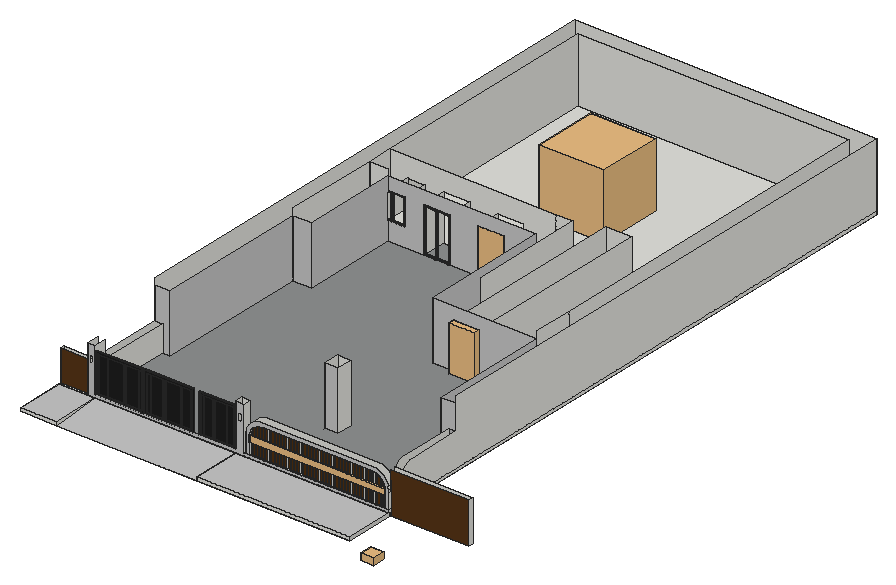
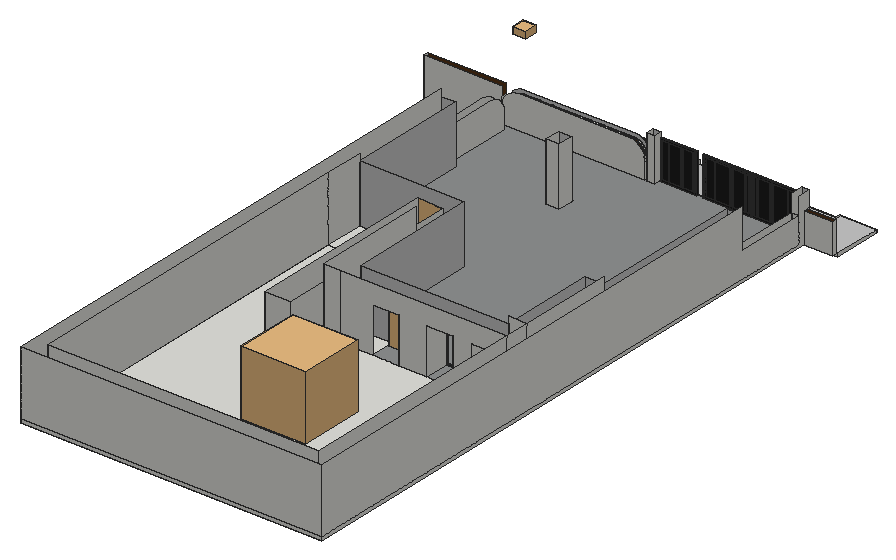
# SketchUp Ruby script. Lengths in inches.
U = 1.inch
M = Sketchup.active_model
def pt(a) = Geom::Point3d.new(a.map { |v| v * U })
def face(e, loops, mat)
  f = e.add_face(loops[0].map { |a| pt(a) })
  loops[1..].each { |l| e.add_face(l.map { |a| pt(a) }).erase! }
  f.material = f.back_material = mat if mat
  f
end
# faces: each face lists its corners as indices into pts; further lists are holes
def faces(e, pts, list, mat = nil) = list.each { |f| face(e, (f[0].is_a?(Array) ? f : [f]).map { |l| l.map { |i| pts[i] } }, mat) }
# xy, xz, yz: faces in a plane at the given z, y or x. An outline is a flat list of corners, or four numbers for a rectangle; further outlines are holes
def ring(l) = l.size == 4 ? [[l[0], l[1]], [l[2], l[1]], [l[2], l[3]], [l[0], l[3]]] : l.each_slice(2).to_a
def flat(e, list, mat, &to3) = list.each { |f| face(e, (f[0].is_a?(Array) ? f : [f]).map { |l| ring(l).map { |u, v| to3.(u, v) } }, mat) }
def xy(e, z, list, mat = nil) = flat(e, list, mat) { |x, y| [x, y, z] }
def xz(e, y, list, mat = nil) = flat(e, list, mat) { |x, z| [x, y, z] }
def yz(e, x, list, mat = nil) = flat(e, list, mat) { |y, z| [x, y, z] }
def lines(e, pts, list) = list.each { |a, b| e.add_line(pt(pts[a]), pt(pts[b])) }
# prism: a flat outline (further loops are holes) pulled along v
def prism(e, loops, v, mat = nil)
  f = face(e, loops, mat); d = Geom::Vector3d.new(v.map { |x| x * U })
  f.pushpull(f.normal.samedirection?(d) ? d.length : -d.length)
end
def box(e, o, s, mat = nil) = prism(e, [[o, [o[0] + s[0], o[1], o[2]], [o[0] + s[0], o[1] + s[1], o[2]], [o[0], o[1] + s[1], o[2]]]], [0, 0, s[2]], mat)
def at(x, y, z, deg = 0) = Geom::Transformation.translation(pt([x, y, z])) * Geom::Transformation.rotation(ORIGIN, Z_AXIS, deg.degrees)
def axes(o, x, y, z) = Geom::Transformation.new([*x, 0, *y, 0, *z, 0, *pt(o).to_a, 1])
def part(name) = M.definitions.add(name)
# library, detail: a bought-in or finely detailed component or shape, given as its bounding box
def library(name, o, s) = part(name).tap { |d| box(d.entities, o, s) }
def detail(e, o, s) = box(e.add_group.entities, o, s)
def put(e, d, t, mat = nil) = e.add_instance(d, t).tap { |i| i.material = mat if mat }
def group(e, t, mat = nil) = e.add_group.tap { |g| g.transformation = t; g.material = mat if mat }.entities
root = M.entities
M.materials.add("Wine2").color = [0, 0, 0]
M.materials["Wine2"].alpha = 0
M.materials.add("[0130_Gainsboro]").color = [39, 45, 50]
M.materials.add("[Blacktop Old 02]").color = [143, 145, 145]
M.materials.add("[Color M02]").color = [198, 198, 198]
M.materials.add("[Color M08]1").color = [30, 30, 30]
M.materials.add("[Wood Floor Dark]").color = [86, 53, 23]
M.materials.add("[Wood Square Tile 02]").color = [81, 47, 16]
c1 = library("door (1)",[38.93,25.48,0],[40,9.94,82.68])
c2 = part("Framed glazing panel")
xy(c2.entities,0,[[0,-0.98,43.07,0],[0,0,43.07,1.4]],"[0130_Gainsboro]")
xy(c2.entities,0.3,[[0.3,-1.43,42.77,-0.98]],"[0130_Gainsboro]")
xy(c2.entities,2.95,[[2.95,-1.43,40.12,-0.63],[2.95,-0.63,40.12,0],[2.95,0,40.12,0.64],[2.95,0.64,40.12,1.4]],"[0130_Gainsboro]")
xy(c2.entities,3.54,[[3.54,-0.63,39.53,0],[3.54,0,39.53,0.64]],"[0130_Gainsboro]")
xy(c2.entities,111.8125,[[3.54,-0.63,39.53,0],[3.54,0,39.53,0.64]],"[0130_Gainsboro]")
xy(c2.entities,112.4,[[2.95,-1.43,40.12,-0.63],[2.95,-0.63,40.12,0],[2.95,0,40.12,0.64],[2.95,0.64,40.12,1.4]],"[0130_Gainsboro]")
xy(c2.entities,115.05,[[0.3,-1.43,42.77,-0.98]],"[0130_Gainsboro]")
xy(c2.entities,115.35,[[0,-0.98,43.07,0],[0,0,43.07,1.4]],"[0130_Gainsboro]")
xz(c2.entities,-1.43,[[[0.3,0.3,42.77,115.05],[2.95,2.95,40.12,112.4]]],"[0130_Gainsboro]")
xz(c2.entities,-0.98,[[[0,0,43.07,115.35],[0.3,0.3,42.77,115.05]]],"[0130_Gainsboro]")
xz(c2.entities,-0.63,[[[2.95,2.95,40.12,112.4],[3.54,3.54,39.53,111.8125]]],"[0130_Gainsboro]")
xz(c2.entities,0,[[3.54,3.54,39.53,111.8125]],"Wine2")
xz(c2.entities,0,[[[0,0,43.07,115.35],[2.95,2.95,40.12,112.4]],[[2.95,2.95,40.12,112.4],[3.54,3.54,39.53,111.8125]]],"[0130_Gainsboro]")
xz(c2.entities,0.64,[[[2.95,2.95,40.12,112.4],[3.54,3.54,39.53,111.8125]]],"[0130_Gainsboro]")
xz(c2.entities,1.4,[[[0,0,43.07,115.35],[2.95,2.95,40.12,112.4]]],"[0130_Gainsboro]")
yz(c2.entities,0,[[-0.98,0,0,115.35],[0,0,1.4,115.35]],"[0130_Gainsboro]")
yz(c2.entities,0.3,[[-1.43,0.3,-0.98,115.05]],"[0130_Gainsboro]")
yz(c2.entities,2.95,[[-1.43,2.95,-0.63,112.4],[-0.63,2.95,0,112.4],[0,2.95,0.64,112.4],[0.64,2.95,1.4,112.4]],"[0130_Gainsboro]")
yz(c2.entities,3.54,[[-0.63,3.54,0,111.8125],[0,3.54,0.64,111.8125]],"[0130_Gainsboro]")
yz(c2.entities,39.53,[[-0.63,3.54,0,111.8125],[0,3.54,0.64,111.8125]],"[0130_Gainsboro]")
yz(c2.entities,40.12,[[-1.43,2.95,-0.63,112.4],[-0.63,2.95,0,112.4],[0,2.95,0.64,112.4],[0.64,2.95,1.4,112.4]],"[0130_Gainsboro]")
yz(c2.entities,42.77,[[-1.43,0.3,-0.98,115.05]],"[0130_Gainsboro]")
yz(c2.entities,43.07,[[-0.98,0,0,115.35],[0,0,1.4,115.35]],"[0130_Gainsboro]")
c3 = part("Group\#1")
put(c3.entities,c2,axes([45.29,1.43,0],[1.05148,0,0],[0,1,0],[0,0,1]))
put(c3.entities,c2,axes([0,1.43,0],[1.05148,0,0],[0,1,0],[0,0,1]))
c4 = part("Group\#102")
g1 = group(c4.entities,at(0,0,0))
prism(g1,[[[0,3,72],[70.5,3,72],[70.5,3,0],[0,3,0]],[[67.5,3,3],[67.5,3,69],[3,3,69],[3,3,3]]],[0,-3,0])
c5 = part("Group\#135")
box(c5.entities,[0,0,0],[0.5,1,66])
c6 = part("Group\#148")
box(c6.entities,[0,-1,0],[5.5,1,66])
box(c6.entities,[50.84,-1,0],[13.66,1,66])
box(c6.entities,[28.06,-1,0],[22.28,1,66])
box(c6.entities,[24.66,-1,0],[2.9,1,66])
box(c6.entities,[6,-1,0],[18.16,1,66])
c7 = part("Entrance gate assembly")
g2 = group(c7.entities,at(70.5,0,0),"[Color M08]1")
put(g2,c4,axes([70.5,0,0],[-1,0,0],[0,1,0],[0,0,1]))
g3 = group(g2,at(3,2,3))
g4 = group(g3,at(0,-1,0))
box(g4,[0,0,0],[5.5,1,66])
box(g4,[50.84,0,0],[13.66,1,66])
box(g4,[28.06,0,0],[22.28,1,66])
box(g4,[24.66,0,0],[2.9,1,66])
box(g4,[6,0,0],[18.16,1,66])
put(g3,c5,axes([50.34,0,0],[1,0,0],[0,-1,0],[0,0,1]))
put(g3,c5,axes([24.16,0,0],[1,0,0],[0,-1,0],[0,0,1]))
put(g3,c5,axes([27.56,0,0],[1,0,0],[0,-1,0],[0,0,1]))
put(g3,c5,axes([5.5,0,0],[1,0,0],[0,-1,0],[0,0,1]))
g5 = group(c7.entities,at(70.5,0,0),"[Color M08]1")
put(g5,c4,at(-70.5,0,0))
g6 = group(g5,at(-3,2,3,-180))
put(g6,c6,at(0,1,0))
put(g6,c5,at(50.34,0,0))
put(g6,c5,at(24.16,0,0))
put(g6,c5,at(27.56,0,0))
put(g6,c5,at(5.5,0,0))
g7 = group(c7.entities,at(150,0,0),"[Color M08]1")
put(g7,c4,axes([54,0,0],[-0.76596,0,0],[0,1,0],[0,0,1]))
g8 = group(g7,at(2.3,2,3))
put(g8,c6,axes([0,-1,0],[0.76596,0,0],[0,-1,0],[0,0,1]))
put(g8,c5,axes([38.55,0,0],[0.76596,0,0],[0,-1,0],[0,0,1]))
put(g8,c5,axes([18.5,0,0],[0.76596,0,0],[0,-1,0],[0,0,1]))
put(g8,c5,axes([21.11,0,0],[0.76596,0,0],[0,-1,0],[0,0,1]))
put(g8,c5,axes([4.22,0,0],[0.76596,0,0],[0,-1,0],[0,0,1]))
c8 = library("Omni Light",[-12,-12,-12],[24,24,24])
c9 = library("Mesh Light\#1",[-0.5,-0.5,-0.1],[1,1,0.2])
c10 = library("Dome Light",[-12,-12,0],[24,24,12])
xy(root,-12.28,[[0,0,326.57,89.5625],[326.57,0,609.5625,89.5625],[610.25,94.125,754.3125,104.0625]])
xy(root,-6,[[0,89.5625,52.9375,94.125],[52.9375,89.5625,52.9375,94.125,0,94.125,0,101.45,52.9375,101.45,52.9375,1217.1875,610.25,1217.1875,610.25,89.5625]])
xy(root,-6,[[0,0,66.8125,89.5625],[326.57,0,610.25,89.5625]],"[Color M02]")
xy(root,0,[[352.65,89.5625,354.44,92.0625],[354.44,89.5625,357.5,92.8125],[357.5,89.5625,361.83,92.0625],[361.83,89.5625,367.13,92.8125],[367.13,89.5625,373.05,92.0625],
  [373.05,89.5625,378.96,92.8125],[378.96,89.5625,384.88,92.0625],[384.88,89.5625,390.79,92.8125],[390.79,89.5625,396.71,92.0625],[396.71,89.5625,402.625,92.8125],
  [402.625,89.5625,408.54,92.0625],[408.54,89.5625,414.45,92.8125],[414.45,89.5625,420.37,92.0625],[420.37,89.5625,426.28,92.8125],[426.28,89.5625,432.2,92.0625],
  [432.2,89.5625,438.11,92.8125],[438.11,89.5625,444.03,92.0625],[444.03,89.5625,449.94,92.8125],[449.94,89.5625,455.86,92.0625],[455.86,89.5625,461.77,92.8125],
  [461.77,89.5625,467.6875,92.0625],[467.6875,89.5625,473.6,92.8125],[473.6,89.5625,479.52,92.0625],[479.52,89.5625,485.43,92.8125],[485.43,89.5625,491.35,92.0625],
  [491.35,89.5625,497.26,92.8125],[497.26,89.5625,503.18,92.0625],[503.18,89.5625,509.09,92.8125],[509.09,89.5625,515,92.0625],[515,89.5625,520.92,92.8125],
  [520.92,89.5625,526.83,92.0625],[526.83,89.5625,532.75,92.8125],[532.75,89.5625,538.66,92.0625],[538.66,89.5625,544.58,92.8125],[544.58,89.5625,550.49,92.0625],
  [550.49,89.5625,556.41,92.8125],[556.41,89.5625,562.32,92.0625],[562.32,89.5625,568.24,92.8125],[568.24,89.5625,572.45,92.0625],[572.45,89.5625,576.66,92.8125],
  [576.66,89.5625,581.24,92.0625],[581.24,89.5625,586.78,92.8125],[586.78,89.5625,592.76,92.0625],[592.76,89.5625,595.36,92.8125],[595.36,89.5625,599.57,92.0625],
  [599.57,89.5625,603.11,92.0625],[52.9375,113,66.86,113,66.86,244.9375,80.78,244.9375,80.78,1189.34,582.4,1189.34,582.4,244.9375,596.33,244.9375,596.33,115.8125,610.25,115.8125,610.25,1217.1875,52.9375,1217.1875],[388.8,467.53,427.3,467.53,427.3,539.85,420.8,539.85,420.8,752.85,329.63,752.85,329.63,706.78,388.8,706.78],[475.3,467.53,582.4,539.85],[420.8,539.85,427.3,539.85,427.3,820.03,475.3,820.03,475.3,539.85,582.4,539.85,582.4,1189.34,80.78,1189.34,80.78,752.85,420.8,752.85],
  [80.78,706.78,181,752.85],[229,706.78,281.63,752.85]])
xy(root,0,[[[66.86,89.5625,326.57,89.5625,326.57,104.75,341.76,104.75,341.76,89.5625,345.52,89.5625,345.52,104.0625,610.25,104.0625,610.25,115.8125,596.33,115.8125,596.33,244.9375,582.4,244.9375,582.4,467.53,475.3,467.53,475.3,820.03,427.3,820.03,427.3,467.53,388.8,467.53,388.8,706.78,329.63,706.78,329.63,752.85,281.63,752.85,281.63,706.78,229,706.78,229,752.85,181,752.85,181,706.78,115.1,706.78,115.1,529.39,80.78,529.39,80.78,244.9375,66.86,244.9375],[388.4375,219.25,412.5,248.6]]],"[Blacktop Old 02]")
xy(root,34.97,[[115.1,706.78,146.03,752.85]])
xz(root,0,[[0,-12.28,66.8125,-6],[326.57,-12.28,609.5625,-12.28,610.25,-6,326.57,-6]])
xz(root,89.5625,[[0,-12.28,326.57,-6],[326.57,-12.28,326.57,-6,610.25,-6,609.5625,-12.28]])
xz(root,89.5625,[[[52.9375,-6,610.25,-6,610.25,0,341.76,0,341.76,79.6875,326.57,79.6875,326.57,0,66.86,0,66.86,79.6875,52.9375,79.6875],[56.17,49.42,62.99,61.98],[330.61,49.42,337.42,61.98]],[345.52,0,352.65,0,352.65,30.59,352.85,33.66,353.45,36.66,354.44,39.57,355.8,42.32,357.5,44.875,359.52,47.18,361.83,49.2,364.38,50.91,367.13,52.27,370.04,53.25,373.05,53.85,376.11,54.05,576.66,54.05,580.11,53.82,581.24,53.6,583.5,53.15,586.78,52.04,589.88,50.51,592.76,48.58,595.36,46.3,597.65,43.7,599.57,40.82,601.1,37.72,602.21,34.44,602.89,31.05,603.11,27.59,603.11,0,610.25,0,610.25,27.59,609.96,31.98,609.11,36.29,607.69,40.45,605.75,44.39,603.31,48.04,600.41,51.35,597.11,54.25,593.45,56.6875,589.51,58.63,585.35,60.04,581.04,60.9,576.66,61.1875,376.11,61.1875,372.12,60.93,368.19,60.15,364.4,58.86,360.8125,57.09,357.49,54.87,354.48,52.23,351.84,49.22,349.62,45.89,347.85,42.3,346.56,38.51,345.78,34.59,345.52,30.59]],"[Color M02]")
xz(root,92.0625,[[352.65,0,354.44,0,354.44,39.57,353.45,36.66,352.85,33.66,352.65,30.59],[357.5,0,361.83,0,361.83,49.2,359.52,47.18,357.5,44.875],[367.13,0,373.05,0,373.05,53.85,370.04,53.25,367.13,52.27],[378.96,0,384.88,54.05],[390.79,0,396.71,54.05],
  [402.625,0,408.54,54.05],[414.45,0,420.37,54.05],[426.28,0,432.2,54.05],[438.11,0,444.03,54.05],[449.94,0,455.86,54.05],
  [461.77,0,467.6875,54.05],[473.6,0,479.52,54.05],[485.43,0,491.35,54.05],[497.26,0,503.18,54.05],[509.09,0,515,54.05],
  [520.92,0,526.83,54.05],[532.75,0,538.66,54.05],[544.58,0,550.49,54.05],[556.41,0,562.32,54.05],[568.24,0,572.45,54.05],
  [576.66,0,581.24,0,581.24,53.6,580.11,53.82,576.66,54.05],[586.78,0,592.76,0,592.76,48.58,589.88,50.51,586.78,52.04],[595.36,0,599.57,0,599.57,40.82,597.65,43.7,595.36,46.3],[599.57,0,603.11,0,603.11,27.59,602.89,31.05,602.21,34.44,601.1,37.72,599.57,40.82]],"[Wood Square Tile 02]")
xz(root,92.8125,[[354.44,0,357.5,0,357.5,44.875,355.8,42.32,354.44,39.57],[361.83,0,367.13,0,367.13,52.27,364.38,50.91,361.83,49.2],[373.05,0,378.96,0,378.96,54.05,376.11,54.05,373.05,53.85],[384.88,0,390.79,54.05],[396.71,0,402.625,54.05],
  [408.54,0,414.45,54.05],[420.37,0,426.28,54.05],[432.2,0,438.11,54.05],[444.03,0,449.94,54.05],[455.86,0,461.77,54.05],
  [467.6875,0,473.6,54.05],[479.52,0,485.43,54.05],[491.35,0,497.26,54.05],[503.18,0,509.09,54.05],[515,0,520.92,54.05],
  [526.83,0,532.75,54.05],[538.66,0,544.58,54.05],[550.49,0,556.41,54.05],[562.32,0,568.24,54.05],[572.45,0,576.66,54.05],
  [581.24,0,586.78,0,586.78,52.04,583.5,53.15,581.24,53.6],[592.76,0,595.36,0,595.36,46.3,592.76,48.58]],"[Wood Square Tile 02]")
xz(root,94.125,[[610.25,-12.28,754.3125,63.75],[0,-6,52.9375,50.9375]],"[Wood Floor Dark]")
xz(root,101.45,[[0,-6,52.9375,50.9375]])
xz(root,104.0625,[[610.25,-12.28,754.3125,63.75],[345.52,0,345.52,30.59,345.78,34.59,346.56,38.51,347.85,42.3,349.62,45.89,351.84,49.22,354.48,52.23,357.49,54.87,360.8125,57.09,364.4,58.86,368.19,60.15,372.12,60.93,376.11,61.1875,576.66,61.1875,581.04,60.9,585.35,60.04,589.51,58.63,593.45,56.6875,597.11,54.25,600.41,51.35,603.31,48.04,605.75,44.39,607.69,40.45,609.11,36.29,609.96,31.98,610.25,27.59,610.25,0]])
xz(root,104.75,[[326.57,0,341.76,79.6875]])
xz(root,113,[[52.9375,0,66.86,48]])
xz(root,115.8125,[[596.33,0,610.25,30.59]])
xz(root,219.25,[[388.4375,0,412.5,107.6875]],"[Color M02]")
xz(root,244.9375,[[66.86,0,80.78,0,80.78,107.6875,52.9375,107.6875,52.9375,48,66.86,48],[582.4,0,596.33,0,596.33,61.1875,610.25,61.1875,610.25,107.6875,582.4,107.6875]],"[Color M02]")
xz(root,248.6,[[388.4375,0,412.5,107.6875]])
xz(root,467.53,[[388.8,0,427.3,0,427.3,84,475.3,84,475.3,0,582.4,0,582.4,107.6875,388.8,107.6875]],"[Color M02]")
xz(root,529.39,[[80.78,0,115.1,107.6875]],"[Color M02]")
xz(root,706.78,[[80.78,0,115.1,120]])
xz(root,706.78,[[115.1,0,181,0,181,84,229,84,229,0,281.63,0,281.63,84,329.63,84,329.63,0,388.8,0,388.8,107.6875,115.1,107.6875,115.1,84,146.03,84,146.03,34.97,115.1,34.97]],"[Color M02]")
xz(root,752.85,[[[80.78,0,80.78,120,388.8,120,388.8,0,329.63,0,329.63,84,281.63,84,281.63,0,229,0,229,84,181,84,181,0],[115.1,34.97,146.03,84]],[388.8,0,420.8,120]])
xz(root,820.03,[[427.3,0,475.3,84]])
xz(root,1189.34,[[80.78,0,582.4,120]])
xz(root,1217.1875,[[52.9375,-6,610.25,0],[52.9375,0,610.25,120]])
yz(root,0,[[0,-12.28,89.5625,-6],[94.125,-6,101.45,50.9375]])
yz(root,52.9375,[[101.45,-6,101.45,50.9375,89.5625,50.9375,89.5625,79.6875,113,79.6875,113,0,1217.1875,0,1217.1875,-6],[89.5625,-6,94.125,50.9375],[113,0,113,48,244.9375,48,244.9375,120,1217.1875,120,1217.1875,0]])
yz(root,66.8125,[[0,-12.28,89.5625,-6,0,-6]])
yz(root,66.86,[[89.5625,0,113,79.6875],[113,0,244.9375,48]])
yz(root,80.78,[[529.39,0,706.78,120],[706.78,0,752.85,120],[752.85,0,1189.34,120]])
yz(root,80.78,[[244.9375,0,529.39,107.6875]],"[Color M02]")
yz(root,115.1,[[706.78,34.97,752.85,84]])
yz(root,115.1,[[529.39,0,706.78,107.6875]],"[Color M02]")
yz(root,146.03,[[706.78,34.97,752.85,84]])
yz(root,181,[[706.78,0,752.85,84]])
yz(root,229,[[706.78,0,752.85,84]])
yz(root,281.63,[[706.78,0,752.85,84]])
yz(root,326.57,[[0,-12.28,0,-6,89.5625,-6],[89.5625,0,104.75,79.6875]])
yz(root,341.76,[[89.5625,0,104.75,79.6875]])
yz(root,345.52,[[89.5625,0,104.0625,30.59]])
yz(root,354.44,[[92.0625,0,92.8125,39.57]])
yz(root,357.5,[[92.0625,0,92.8125,44.875]])
yz(root,361.83,[[92.0625,0,92.8125,49.2]])
yz(root,367.13,[[92.0625,0,92.8125,52.27]])
yz(root,373.05,[[92.0625,0,92.8125,52.27]])
yz(root,378.96,[[92.0625,0,92.8125,52.27]])
yz(root,384.88,[[92.0625,0,92.8125,52.27]])
yz(root,388.4375,[[219.25,0,248.6,107.6875]])
yz(root,388.8,[[467.53,0,706.78,107.6875]],"[Color M02]")
yz(root,390.79,[[92.0625,0,92.8125,52.27]])
yz(root,396.71,[[92.0625,0,92.8125,52.27]])
yz(root,402.625,[[92.0625,0,92.8125,52.27]])
yz(root,408.54,[[92.0625,0,92.8125,52.27]])
yz(root,412.5,[[219.25,0,248.6,107.6875]])
yz(root,414.45,[[92.0625,0,92.8125,52.27]])
yz(root,420.37,[[92.0625,0,92.8125,52.27]])
yz(root,420.8,[[539.85,0,752.85,120]])
yz(root,426.28,[[92.0625,0,92.8125,52.27]])
yz(root,427.3,[[467.53,0,820.03,84]])
yz(root,432.2,[[92.0625,0,92.8125,52.27]])
yz(root,438.11,[[92.0625,0,92.8125,52.27]])
yz(root,444.03,[[92.0625,0,92.8125,52.27]])
yz(root,449.94,[[92.0625,0,92.8125,52.27]])
yz(root,455.86,[[92.0625,0,92.8125,52.27]])
yz(root,461.77,[[92.0625,0,92.8125,52.27]])
yz(root,467.6875,[[92.0625,0,92.8125,52.27]])
yz(root,473.6,[[92.0625,0,92.8125,52.27]])
yz(root,475.3,[[467.53,0,820.03,84]])
yz(root,479.52,[[92.0625,0,92.8125,52.27]])
yz(root,485.43,[[92.0625,0,92.8125,52.27]])
yz(root,491.35,[[92.0625,0,92.8125,52.27]])
yz(root,497.26,[[92.0625,0,92.8125,52.27]])
yz(root,503.18,[[92.0625,0,92.8125,52.27]])
yz(root,509.09,[[92.0625,0,92.8125,52.27]])
yz(root,515,[[92.0625,0,92.8125,52.27]])
yz(root,520.92,[[92.0625,0,92.8125,52.27]])
yz(root,526.83,[[92.0625,0,92.8125,52.27]])
yz(root,532.75,[[92.0625,0,92.8125,52.27]])
yz(root,538.66,[[92.0625,0,92.8125,52.27]])
yz(root,544.58,[[92.0625,0,92.8125,52.27]])
yz(root,550.49,[[92.0625,0,92.8125,50.58]])
yz(root,556.41,[[92.0625,0,92.8125,52.27]])
yz(root,562.32,[[92.0625,0,92.8125,52.27]])
yz(root,568.24,[[92.0625,0,92.8125,52.27]])
yz(root,572.45,[[92.0625,0,92.8125,54.05]])
yz(root,576.66,[[92.0625,0,92.8125,54.05]])
yz(root,581.24,[[92.0625,0,92.8125,53.6]])
yz(root,582.4,[[467.53,0,539.85,120],[539.85,0,1189.34,120]])
yz(root,582.4,[[244.9375,0,467.53,107.6875]],"[Color M02]")
yz(root,586.78,[[92.0625,0,92.8125,52.04]])
yz(root,592.76,[[92.0625,0,92.8125,48.58]])
yz(root,595.36,[[92.0625,0,92.8125,46.3]])
yz(root,596.33,[[115.8125,0,115.8125,30.59,116.07,34.59,116.85,38.51,118.14,42.3,119.91,45.89,122.13,49.22,124.77,52.23,127.78,54.87,131.11,57.09,134.7,58.86,138.49,60.15,142.41,60.93,146.41,61.1875,244.9375,61.1875,244.9375,0]])
yz(root,610.25,[[94.125,-12.28,104.0625,-6],[89.5625,-6,94.125,0],[94.125,-6,104.0625,0],[104.0625,-6,1217.1875,0],[89.5625,0,94.125,27.59],
  [94.125,0,104.0625,27.59],[115.8125,0,1217.1875,0,1217.1875,120,244.9375,120,244.9375,61.1875,146.41,61.1875,142.41,60.93,138.49,60.15,134.7,58.86,131.11,57.09,127.78,54.87,124.77,52.23,122.13,49.22,119.91,45.89,118.14,42.3,116.85,38.51,116.07,34.59,115.8125,30.59],[94.125,27.59,104.0625,45.67]])
yz(root,754.3125,[[94.125,-12.28,104.0625,63.75]])
p = [[326.57,89.5625,-6],[66.8125,89.5625,-6],[66.8125,0,-12.28],[326.57,0,-12.28],[609.5625,89.5625,-12.28],[610.25,89.5625,-6],
  [610.25,0,-6],[609.5625,0,-12.28],[609.96,104.0625,31.98],[609.96,89.5625,31.98],[610.25,89.5625,27.59],[610.25,94.125,27.59],
  [610.25,104.0625,27.59],[345.52,104.0625,30.59],[345.52,89.5625,30.59],[345.78,89.5625,34.59],[345.78,104.0625,34.59],[610.25,115.8125,30.59],
  [610.25,116.07,34.59],[596.33,116.07,34.59],[596.33,115.8125,30.59],[609.11,104.0625,36.29],[609.11,89.5625,36.29],[346.56,89.5625,38.51],
  [346.56,104.0625,38.51],[610.25,116.85,38.51],[596.33,116.85,38.51],[388.4375,215.23,0],[388.4375,219.25,0]]
faces(root,p,[[0,1,2,3]],"[Color M02]")
faces(root,p,[[4,5,6,7],[8,9,10,11,12],[13,14,15,16],[17,18,19,20],[21,22,9,8],[16,15,23,24],[18,25,26,19]])
lines(root,p,[[27,28]])
put(root,c1,axes([234.92,681.3,-0.33],[1.2,0,0],[0,1,0],[0,0,1.02]))
put(root,c1,axes([380.59,432.12,-0.33],[1.2,0,0],[0,1,0],[0,0,1.02]))
put(root,c3,axes([181.25,708.34,0],[0.52722,0,0],[0,-0.55,0],[0,0,0.72819]))
put(root,c7,axes([68.67,89.5625,0],[1.26423,0,0],[0,1,0],[0,0,1]))
put(root,c8,axes([301.53,957.45,60],[5,0,0],[0,5,0],[0,0,5]))
g9 = group(root,at(352.65,89.5625,0))
xy(g9,54.05,[[23.46,0,26.31,3.25],[26.31,0,32.22,2.5],[32.22,0,38.14,3.25],[38.14,0,44.05,2.5],[44.05,0,49.97,3.25],
  [49.97,0,55.88,2.5],[55.88,0,61.8,3.25],[61.8,0,67.71,2.5],[67.71,0,73.63,3.25],[73.63,0,79.54,2.5],
  [79.54,0,85.46,3.25],[85.46,0,91.37,2.5],[91.37,0,97.29,3.25],[97.29,0,103.2,2.5],[103.2,0,109.12,3.25],
  [109.12,0,115.03,2.5],[115.03,0,120.95,3.25],[120.95,0,126.86,2.5],[126.86,0,132.78,3.25],[132.78,0,138.69,2.5],
  [138.69,0,144.61,3.25],[144.61,0,150.52,2.5],[150.52,0,156.4375,3.25],[156.4375,0,162.35,2.5],[162.35,0,168.27,3.25],
  [168.27,0,174.18,2.5],[174.18,0,180.1,3.25],[180.1,0,186.01,2.5],[186.01,0,191.92,3.25],[191.92,0,197.84,2.5],
  [197.84,0,203.75,3.25],[203.75,0,209.67,2.5],[209.67,0,215.58,3.25],[215.58,0,219.79,2.5],[219.79,0,224,3.25]])
yz(g9,0,[[0,0,2.5,30.59]])
yz(g9,250.46,[[0,0,2.5,27.59]])
p = [[250.23,2.5,31.05],[250.46,2.5,27.59],[250.46,0,27.59],[250.23,0,31.05],[0,2.5,30.59],[0.2,2.5,33.66],
  [0.2,0,33.66],[0,0,30.59],[249.56,2.5,34.44],[249.56,0,34.44],[0.8,2.5,36.66],[0.8,0,36.66],
  [248.45,2.5,37.72],[248.45,0,37.72],[1.79,2.5,39.57],[1.79,0,39.57],[246.91,2.5,40.82],[246.91,0,40.82],
  [3.14,3.25,42.32],[3.14,0,42.32],[1.79,3.25,39.57],[244.99,2.5,43.7],[244.99,0,43.7],[4.85,3.25,44.875],
  [4.85,2.5,44.875],[4.85,0,44.875],[242.71,2.5,46.3],[242.71,0,46.3],[6.87,2.5,47.18],[6.87,0,47.18],
  [242.71,3.25,46.3],[240.11,0,48.58],[240.11,2.5,48.58],[240.11,3.25,48.58],[9.18,2.5,49.2],[9.18,0,49.2],
  [237.23,2.5,50.51],[237.23,0,50.51],[11.73,3.25,50.91],[11.73,0,50.91],[9.18,3.25,49.2],[234.125,2.5,52.04],
  [234.125,0,52.04],[14.48,3.25,52.27],[14.48,2.5,52.27],[14.48,0,52.27],[234.125,3.25,52.04],[230.85,0,53.15],
  [230.85,3.25,53.15],[17.39,2.5,53.25],[17.39,0,53.25],[228.58,0,53.6],[228.58,2.5,53.6],[228.58,3.25,53.6],
  [20.4,2.5,53.85],[20.4,0,53.85],[227.46,2.5,53.82],[227.46,0,53.82],[23.46,3.25,54.05],[23.46,0,54.05],
  [20.4,3.25,53.85],[224,2.5,54.05],[224,0,54.05]]
faces(g9,p,[[0,1,2,3],[4,5,6,7],[8,0,3,9],[5,10,11,6],[12,8,9,13],[10,14,15,11],[16,12,13,17],[18,19,15,14,20],
  [21,16,17,22],[23,24,25,19,18],[26,21,22,27],[24,28,29,25],[30,26,27,31,32,33],[28,34,35,29],[36,32,31,37],[38,39,35,34,40],
  [41,36,37,42],[43,44,45,39,38],[46,41,42,47,48],[44,49,50,45],[48,47,51,52,53],[49,54,55,50],[56,52,51,57],[58,59,55,54,60],
  [61,56,57,62]])
put(g9,c9,axes([125.23,1.625,27.03],[251.4591,0,0],[0,4.25,0],[0,0,55.0506]))
put(root,c10,at(718.2,-83.32,30.42))
put(root,c3,axes([98.28,708.34,34.97],[0.52722,0,0],[0,-0.55,0],[0,0,0.42503]))
